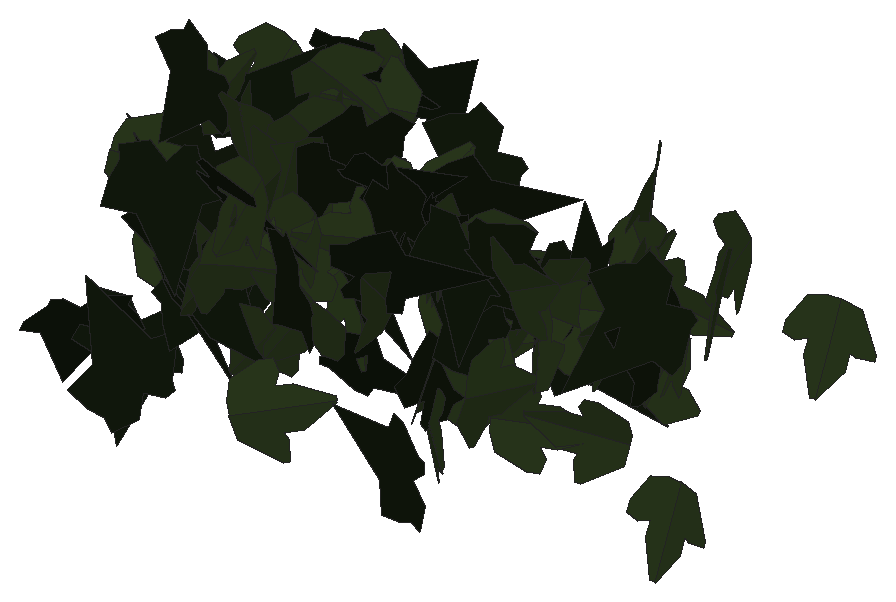
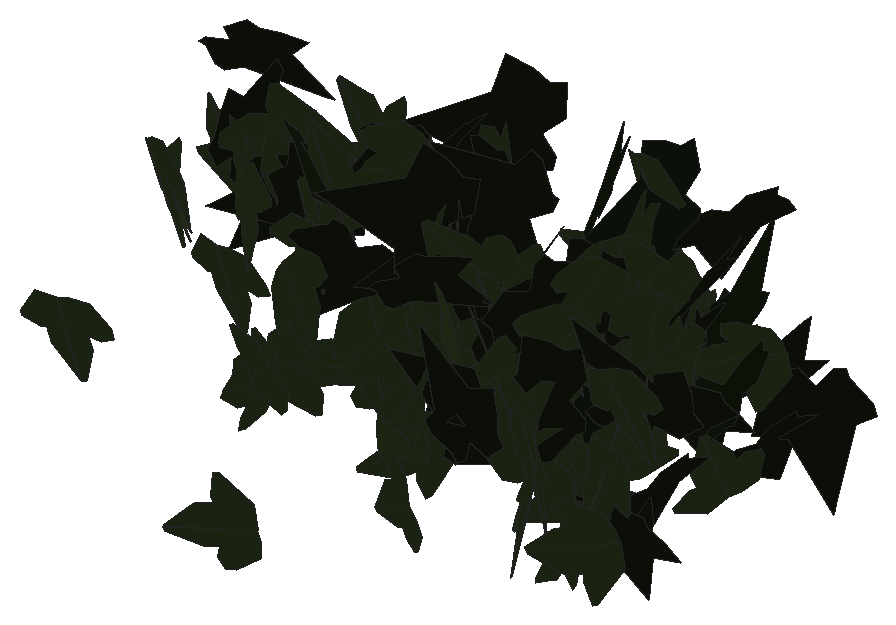
# SketchUp Ruby script. Lengths in inches.
U = 1.inch
M = Sketchup.active_model
def pt(a) = Geom::Point3d.new(a.map { |v| v * U })
def face(e, loops, mat)
  f = e.add_face(loops[0].map { |a| pt(a) })
  loops[1..].each { |l| e.add_face(l.map { |a| pt(a) }).erase! }
  f.material = f.back_material = mat if mat
  f
end
# faces: each face lists its corners as indices into pts; further lists are holes
def faces(e, pts, list, mat = nil) = list.each { |f| face(e, (f[0].is_a?(Array) ? f : [f]).map { |l| l.map { |i| pts[i] } }, mat) }
# xy, xz, yz: faces in a plane at the given z, y or x. An outline is a flat list of corners, or four numbers for a rectangle; further outlines are holes
def ring(l) = l.size == 4 ? [[l[0], l[1]], [l[2], l[1]], [l[2], l[3]], [l[0], l[3]]] : l.each_slice(2).to_a
def flat(e, list, mat, &to3) = list.each { |f| face(e, (f[0].is_a?(Array) ? f : [f]).map { |l| ring(l).map { |u, v| to3.(u, v) } }, mat) }
def xy(e, z, list, mat = nil) = flat(e, list, mat) { |x, y| [x, y, z] }
def xz(e, y, list, mat = nil) = flat(e, list, mat) { |x, z| [x, y, z] }
def yz(e, x, list, mat = nil) = flat(e, list, mat) { |y, z| [x, y, z] }
def lines(e, pts, list) = list.each { |a, b| e.add_line(pt(pts[a]), pt(pts[b])) }
# prism: a flat outline (further loops are holes) pulled along v
def prism(e, loops, v, mat = nil)
  f = face(e, loops, mat); d = Geom::Vector3d.new(v.map { |x| x * U })
  f.pushpull(f.normal.samedirection?(d) ? d.length : -d.length)
end
def box(e, o, s, mat = nil) = prism(e, [[o, [o[0] + s[0], o[1], o[2]], [o[0] + s[0], o[1] + s[1], o[2]], [o[0], o[1] + s[1], o[2]]]], [0, 0, s[2]], mat)
def at(x, y, z, deg = 0) = Geom::Transformation.translation(pt([x, y, z])) * Geom::Transformation.rotation(ORIGIN, Z_AXIS, deg.degrees)
def axes(o, x, y, z) = Geom::Transformation.new([*x, 0, *y, 0, *z, 0, *pt(o).to_a, 1])
def part(name) = M.definitions.add(name)
# library, detail: a bought-in or finely detailed component or shape, given as its bounding box
def library(name, o, s) = part(name).tap { |d| box(d.entities, o, s) }
def detail(e, o, s) = box(e.add_group.entities, o, s)
def put(e, d, t, mat = nil) = e.add_instance(d, t).tap { |i| i.material = mat if mat }
def group(e, t, mat = nil) = e.add_group.tap { |g| g.transformation = t; g.material = mat if mat }.entities
root = M.entities
M.materials.add("efeu1").color = [18, 25, 13]
M.materials.add("efeu2").color = [43, 57, 29]
c1 = part("ivyleaf_9")
p = [[1.54,2.16,1.25],[1.36,2.04,1.19],[-0.21,0.99,0.68],[-0.71,1.11,0.82],[-0.85,0.86,0.67],[-0.8,0.17,0.21],
  [-0.9,-0.01,0.1],[-0.67,-0.16,-0.02],[-0.08,-0.08,-0.05],[-0.03,-0.6,-0.4],[0.65,-0.88,-0.66],[0.83,-0.6,-0.49],
  [1.29,-0.42,-0.43],[1.8125,-0.07,-0.26],[1.21,0.44,0.15]]
faces(c1.entities,p,[[0,1,2,3,4,5,6,7,8,9,10,11,12,13,14]],"efeu1")
c2 = part("ivyleaf_10")
p = [[0,0.5,-0.03],[-0.0625,2.02,-0.43],[-0.19,2.01,-0.46],[-0.54,1.05,-0.29],[-0.52,0.625,-0.18],[-0.83,0.76,-0.28],
  [-1.16,0.64,-0.33],[-1.15,0.33,-0.24],[-0.77,-0.39,0.02],[-0.3,-0.51,0.16],[0.04,-0.48,0.23],[-0.02,2.01,-0.4375],
  [-0.06,2.01,-0.43],[0.04,-0.49,0.23],[0.67,-0.49,0.14],[1.38,0.36,-0.2],[1.375,0.51,-0.24],[0.81,0.65,-0.19],
  [0.62,0.59,-0.15],[0.6,1.09,-0.28],[0.5,1.23,-0.31]]
faces(c2.entities,p,[[0,1,2,3,4,5,6,7,8,9,10],[11,12,0,13,14,15,16,17,18,19,20]],"efeu2")
put(root,c1,axes([525.73,135.11,155.54],[0.37666,-0.56346,0.39178],[0.22865,-0.31835,-0.67766],[0.64707,0.44048,0.0114]))
put(root,c2,axes([526.19,134.96,153.36],[0.33775,0.58636,-0.33865],[0.14241,0.30846,0.67612],[0.66198,-0.36552,0.02733]))
put(root,c1,axes([526.49,131.96,153.91],[0.23337,0.62056,-0.38436],[-0.13918,-0.3583,-0.66299],[-0.71657,0.2717,0.00359]))
put(root,c2,axes([526.46,137.81,156.6],[0.70776,-0.14583,-0.30515],[-0.29443,0.08256,-0.72236],[0.16641,0.7663,0.01975]))
put(root,c2,axes([526.28,135.94,156.4],[0.05117,0.19029,-0.67696],[0.14044,0.66231,0.19679],[0.68903,-0.14913,0.01016]))
put(root,c2,axes([525.83,134.31,155.91],[-0.14356,-0.14885,-0.75209],[0.73421,0.19361,-0.17847],[0.22074,-0.74078,0.10448]))
put(root,c2,axes([526.39,138.1,155.05],[-0.66717,0.22134,-0.14554],[0.13083,-0.06761,-0.70256],[-0.23034,-0.6795,0.0225]))
put(root,c1,axes([526.29,137.07,154.2],[-0.03514,-0.79581,0.03387],[0.00121,-0.03395,-0.79658],[0.79653,-0.03505,0.0027]))
put(root,c1,axes([526.53,135.75,155.45],[-0.62542,-0.36181,-0.31053],[0.26494,0.16212,-0.72251],[0.39641,-0.67919,-0.00704]))
put(root,c2,axes([526.84,137.6875,154.86],[0.05179,0.09369,-0.70529],[-0.46103,-0.5342,-0.10482],[-0.54191,0.46342,0.02177]))
put(root,c2,axes([526.11,138.74,153.84],[-0.30774,0.05623,-0.71935],[0.7176,-0.05784,-0.31151],[-0.07537,-0.78027,-0.02874]))
put(root,c2,axes([526.68,137.98,154.46],[-0.33118,0.62006,0.1589],[0.0703,-0.14259,0.70295],[0.63623,0.33852,0.00504]))
put(root,c1,axes([526.71,137.6875,153.73],[-0.71609,-0.28278,-0.3521],[0.32978,0.1235,-0.76988],[0.30852,-0.78836,0.00569]))
put(root,c2,axes([526.35,137.02,155.77],[0.23807,-0.32545,0.65801],[0.50385,-0.43064,-0.39529],[0.53388,0.55154,0.07963]))
put(root,c1,axes([526.59,135.45,157.38],[-0.12657,-0.54335,0.52327],[-0.05752,-0.52209,-0.55604],[0.75216,-0.13135,0.04553]))
put(root,c1,axes([526.41,136.85,155.47],[-0.35697,0.12119,0.75407],[0.71327,-0.24468,0.37698],[0.27305,0.79761,0.00107]))
put(root,c2,axes([527.42,137.72,153.65],[0.24405,-0.16605,-0.66016],[-0.53993,0.37987,-0.29515],[0.41456,0.5925,0.00422]))
put(root,c1,axes([526.87,133.15,153.21],[-0.14848,-0.76576,0.05285],[-0.01587,-0.05076,-0.78],[0.76742,-0.14921,-0.0059]))
put(root,c2,axes([527.35,139.04,155.32],[0.34899,-0.44864,-0.39026],[-0.20276,0.33561,-0.56713],[0.55899,0.40183,0.03794]))
put(root,c2,axes([527.43,138.9375,156.24],[-0.11381,-0.59526,0.33256],[-0.04662,-0.32958,-0.60588],[0.68026,-0.12218,0.01412]))
put(root,c2,axes([527.82,137.77,154.49],[-0.47095,-0.11357,0.54585],[-0.50765,-0.20807,-0.48128],[0.23051,-0.69025,0.05527]))
put(root,c2,axes([527.48,135.5,156.73],[-0.73484,0.04403,0.0393],[-0.03958,-0.00361,-0.73613],[-0.04377,-0.73588,0.00596]))
put(root,c2,axes([527.48,138.98,154.92],[-0.33483,0.53964,0.27175],[-0.17377,0.21156,-0.63421],[-0.57867,-0.37578,0.03321]))
put(root,c2,axes([527.47,137.78,153.18],[0.03047,-0.14897,-0.70715],[0.0189,0.7077,-0.14827],[0.72242,-0.01223,0.03371]))
put(root,c1,axes([527.23,136.64,152.72],[-0.34943,0.15803,0.67847],[0.41809,-0.55957,0.34567],[0.55722,0.51896,0.16611]))
put(root,c2,axes([527.51,139.19,155.31],[-0.59921,-0.22011,0.27285],[0.2718,0.04956,0.63688],[-0.22141,0.65654,0.0434]))
put(root,c1,axes([527.08,138.56,156.42],[0.66341,-0.03506,0.43888],[0.43733,-0.03928,-0.6642],[0.0509,0.79447,-0.01347]))
put(root,c2,axes([527.96,139.09,156.48],[0.50985,-0.29969,-0.37154],[-0.31309,0.20041,-0.59128],[0.36033,0.59818,0.01196]))
put(root,c2,axes([528.09,136.21,153.87],[0.43176,-0.20389,0.53418],[-0.48313,0.2279,0.47748],[-0.30579,-0.64795,-0.00015]))
put(root,c1,axes([527.68,132.93,155.23],[0.55391,-0.54398,-0.11808],[0.08585,-0.08111,0.77635],[-0.54999,-0.56052,0.00226]))
put(root,c1,axes([528.06,136.39,155.44],[-0.3816,0.41646,-0.52655],[0.36418,-0.3804,-0.56479],[-0.56398,-0.52742,-0.00842]))
put(root,c1,axes([528.27,131.45,153.125],[-0.46136,-0.60384,0.18477],[0.11557,0.14422,0.75991],[-0.62081,0.4756,0.00415]))
put(root,c2,axes([528.04,137.41,156.07],[-0.06281,-0.44523,-0.52849],[0.05937,0.52523,-0.44954],[0.68848,-0.08591,-0.00945]))
put(root,c2,axes([527.63,136.95,153.6],[0.15666,0.15875,0.68166],[0.39485,0.5567,-0.22039],[-0.57788,0.42341,0.0342]))
put(root,c2,axes([527.87,137.4,157],[-0.51535,-0.23976,-0.514],[0.47284,0.20192,-0.56826],[0.31323,-0.69929,0.01215]))
put(root,c2,axes([528.47,137.875,153.66],[-0.3783,0.42346,0.46618],[-0.30882,0.34922,-0.56783],[-0.54888,-0.48835,-0.00182]))
put(root,c1,axes([528.1,132.43,157.25],[-0.11932,-0.75762,-0.22579],[0.02574,0.22451,-0.76691],[0.79013,-0.12173,-0.00912]))
put(root,c2,axes([528.26,136.81,154.4],[0.61908,0.36942,0.04018],[0.03531,0.01923,-0.72092],[-0.36992,0.62009,-0.00157]))
put(root,c2,axes([528.75,138.28,156.12],[0.13292,0.19344,0.65385],[-0.33366,-0.5625,0.23424],[0.59465,-0.35886,-0.01471]))
put(root,c2,axes([527.94,135.1,154.68],[0.35602,0.15154,0.64477],[0.5863,0.26844,-0.38682],[-0.30813,0.68587,0.00894]))
put(root,c2,axes([528.44,136.35,155.38],[0.05455,0.30482,-0.67747],[-0.08227,-0.67264,-0.30927],[-0.73832,0.09747,-0.01559]))
put(root,c2,axes([528.41,133.25,154.74],[-0.0758,0.11365,0.83409],[0.47877,-0.68301,0.13657],[0.69239,0.48472,-0.00312]))
put(root,c1,axes([528.17,132.82,154.48],[0.45781,-0.56256,0.32268],[0.20926,-0.24572,-0.72527],[0.61385,0.50332,0.00658]))
put(root,c1,axes([528.57,132.77,155],[0.16251,-0.46561,-0.62034],[-0.12427,0.60999,-0.4904],[0.76562,0.19784,0.05207]))
put(root,c2,axes([528.71,135.53,157.05],[-0.37942,-0.41519,-0.37968],[0.26265,0.27427,-0.5624],[0.49755,-0.4614,0.00735]))
put(root,c1,axes([528.65,139.36,155.46],[-0.24925,0.09443,0.71655],[0.50871,-0.51549,0.24489],[0.51339,0.55664,0.10522]))
put(root,c2,axes([529.16,134.7,156.82],[-0.28766,-0.75884,0.09762],[-0.02405,-0.09528,-0.81145],[0.76471,-0.28844,0.01121]))
put(root,c2,axes([529.62,133.51,153.81],[-0.54475,-0.1323,0.46695],[-0.45395,-0.10941,-0.56059],[0.17168,-0.70911,-0.00062]))
put(root,c2,axes([529.07,132.65,155.52],[-0.18011,-0.28273,-0.72286],[0.38507,0.61176,-0.33523],[0.67393,-0.42511,-0.00165]))
put(root,c1,axes([529.54,136.37,156.77],[-0.09222,0.37815,-0.77973],[0.16906,-0.76122,-0.38917],[-0.84994,-0.19245,0.00719]))
put(root,c2,axes([529.18,133.98,156.65],[-0.0628,0.07664,0.88256],[0.4505,-0.75907,0.09797],[0.76278,0.45462,0.0148]))
put(root,c1,axes([529.02,134.82,156.35],[0.18557,0.30961,-0.69755],[0.35331,0.60146,0.36095],[0.67647,-0.39907,0.00284]))
put(root,c2,axes([529.02,137.51,155.06],[-0.00553,0.02222,-0.80273],[0.64831,-0.47358,-0.01758],[-0.47388,-0.64817,-0.01467]))
put(root,c2,axes([529.8,134.24,155.79],[0.64503,-0.3477,-0.28676],[-0.252,0.13685,-0.73278],[0.37366,0.69251,0.00083]))
put(root,c1,axes([529.2,132.51,157.28],[0.78111,-0.2162,0.19855],[0.19335,-0.04571,-0.81045],[0.22086,0.80465,0.00731]))
put(root,c2,axes([529.39,134.41,154.76],[0.43202,0.20004,-0.62224],[0.53966,0.31162,0.47487],[0.36873,-0.69045,0.03404]))
put(root,c2,axes([530.04,132.39,157.39],[0.67732,-0.3914,-0.31063],[-0.26731,0.15825,-0.78227],[0.42217,0.72816,0.00304]))
put(root,c2,axes([530.63,133.37,154.72],[-0.68411,-0.16117,0.54079],[-0.529,-0.11269,-0.70278],[0.19644,-0.86473,-0.00921]))
put(root,c1,axes([530.7,136.16,154.95],[-0.06331,0.2723,0.7111],[-0.24205,0.66935,-0.27786],[-0.72196,-0.24829,0.0308]))
put(root,c1,axes([529.63,137.25,154.41],[0.19437,-0.07367,0.84761],[0.77775,-0.33712,-0.20765],[0.34494,0.80161,-0.00942]))
put(root,c2,axes([530.97,134.86,155.7],[0.05622,0.03281,0.71911],[-0.49015,-0.52652,0.06235],[0.52721,-0.49301,-0.01873]))
put(root,c2,axes([530.9,135.92,156.15],[0.46301,-0.39093,-0.41607],[-0.3309,0.25279,-0.60574],[0.46524,0.56885,-0.01676]))
put(root,c2,axes([530.15,139.28,153.46],[0.32042,-0.11567,0.69432],[0.67291,-0.17348,-0.33944],[0.20651,0.74475,0.02877]))
put(root,c1,axes([530.57,134.89,155.03],[0.56537,-0.36927,-0.42469],[-0.35413,0.23445,-0.67528],[0.4374,0.66712,0.00223]))
put(root,c2,axes([530.53,134.81,154.58],[0.58943,-0.1697,0.4472],[0.42898,-0.12637,-0.61337],[0.21158,0.72901,-0.00222]))
put(root,c2,axes([531.11,137.57,154.77],[0.05845,0.15944,-0.73633],[-0.1167,0.73154,0.14914],[0.7443,0.10218,0.08121]))
put(root,c1,axes([530.59,134.36,153.34],[0.63359,-0.06482,0.47014],[0.46697,-0.05472,-0.63687],[0.08464,0.78706,-0.00556]))
put(root,c1,axes([531.84,137.23,156.71],[-0.55919,-0.43601,0.27616],[-0.2196,-0.16748,-0.70908],[0.46706,-0.60076,-0.00275]))
put(root,c2,axes([531.48,136.34,155.3],[0.5336,-0.55502,-0.01206],[0.01156,-0.00561,0.76991],[-0.55503,-0.53371,0.00445]))
put(root,c1,axes([531.4,132.12,156.05],[-0.03624,-0.32301,0.75298],[0.05393,-0.75302,-0.32043],[0.81756,0.03535,0.05452]))
put(root,c2,axes([531.43,135.43,156.14],[0.5123,0.32592,-0.55248],[0.45205,0.3182,0.60689],[0.45509,-0.68296,0.0191]))
put(root,c1,axes([531.22,134.5,157.02],[0.58662,0.32956,-0.39131],[0.32535,0.21914,0.67229],[0.39482,-0.67024,0.0274]))
put(root,c2,axes([531.79,137.67,153.91],[0.17378,-0.53167,0.51439],[0.15306,-0.49112,-0.55933],[0.72377,0.23152,-0.00523]))
put(root,c2,axes([532.12,135.99,154.32],[0.61286,-0.05358,0.41692],[-0.41608,0.02749,0.61515],[-0.05977,-0.74072,-0.00733]))
put(root,c1,axes([531.96,134.64,155.94],[0.15705,0.21496,0.73889],[0.24435,0.70116,-0.25592],[-0.7297,0.28106,0.07333]))
put(root,c2,axes([531.73,136.44,153.02],[-0.03118,-0.14763,-0.75567],[0.48735,0.58172,-0.13375],[0.59609,-0.48333,0.06983]))
put(root,c2,axes([531.51,130.67,154.16],[0.20551,0.02166,-0.78165],[0.7732,0.11491,0.20648],[0.11663,-0.8,0.0085]))
put(root,c1,axes([531.92,134.18,157.22],[-0.05725,-0.04436,-0.82621],[0.79741,0.21799,-0.06695],[0.22074,-0.79898,0.0276]))
put(root,c1,axes([532.14,134.64,155.95],[0.54878,0.22463,0.5522],[0.50604,0.22122,-0.59289],[-0.31513,0.74642,0.00954]))
put(root,c2,axes([532.49,135.35,156.35],[0.14707,-0.39968,0.69972],[0.40955,-0.57549,-0.4148],[0.69399,0.42432,0.09651]))
put(root,c2,axes([532.72,136.26,154.72],[-0.00258,-0.06448,-0.77656],[0.19562,0.75164,-0.06306],[0.75427,-0.19516,0.0137]))
put(root,c2,axes([532.96,136.34,154.09],[-0.10456,-0.43135,0.57598],[-0.11579,-0.56436,-0.44367],[0.71021,-0.15551,0.01247]))
put(root,c2,axes([532.77,134.19,153.42],[0.32285,-0.76799,0.1296],[-0.04993,0.1196,0.83309],[-0.77724,-0.32669,0.00031]))
put(root,c2,axes([532.82,134.96,154.35],[0.76639,0.1115,0.03958],[-0.03917,-0.00567,0.77445],[0.11164,-0.76739,0.00002]))
put(root,c1,axes([532.72,134.27,153.28],[0.00662,0.03793,0.80643],[0.55066,0.58952,-0.03225],[-0.59037,0.5503,-0.02103]))
put(root,c2,axes([533.24,136.39,155.03],[-0.43748,-0.56914,0.1306],[-0.07998,-0.10325,-0.71785],[0.57843,-0.44473,-0.00048]))
put(root,c2,axes([532.7,134.41,152.7],[-0.07548,0.06886,-0.76785],[0.41704,-0.64524,-0.09886],[-0.64839,-0.42303,0.02579]))
put(root,c1,axes([532.51,135.27,156.77],[0.36655,-0.00786,0.73551],[0.73501,0.03547,-0.36592],[-0.02825,0.82102,0.02286]))
put(root,c2,axes([532.75,134.43,156.38],[0.06314,-0.03133,0.7733],[0.62401,-0.45689,-0.06946],[0.45781,0.62708,-0.01198]))
put(root,c2,axes([533.31,132.45,156.24],[-0.11521,-0.55365,-0.58018],[-0.04052,-0.58136,0.56283],[-0.80093,0.10906,0.05498]))
put(root,c2,axes([533.54,135.1,153.28],[-0.01385,0.59627,0.47066],[-0.02094,-0.47086,0.5959],[0.75935,-0.00211,0.02501]))
put(root,c2,axes([532.91,140.65,152.62],[0.138,0.01796,0.76106],[0.69454,0.31373,-0.13335],[-0.31171,0.70699,0.03983]))
put(root,c1,axes([533.8,132.37,152.79],[0.15673,-0.79501,0.05984],[0.0044,0.06185,0.81015],[-0.79725,-0.15595,0.01623]))
put(root,c1,axes([533.07,131.87,156.97],[0.45293,0.05067,0.6925],[0.6848,0.10406,-0.45551],[-0.11477,0.82089,0.01499]))
put(root,c1,axes([534.01,134.28,155],[-0.1225,-0.79978,0.1421],[0.02146,0.14047,0.80911],[-0.81202,0.12436,-0.00006]))
put(root,c2,axes([534.17,138.42,154.25],[0.11963,-0.23907,0.6877],[-0.2474,0.6421,0.26625],[-0.68474,-0.27376,0.02394]))
put(root,c1,axes([533.87,133.92,156.98],[0.03729,-0.79551,0.19246],[0.0098,-0.19221,-0.79638],[0.8184,0.03855,0.00076]))
put(root,c2,axes([533.7,138.98,154.92],[0.49195,-0.01391,0.55242],[0.55161,-0.0318,-0.49203],[0.03299,0.73904,-0.01077]))
put(root,c2,axes([534.07,134.21,157.15],[-0.56963,-0.02773,-0.54153],[0.54063,0.03134,-0.57029],[0.04169,-0.78533,-0.00364]))
put(root,c1,axes([534.06,133.92,156.89],[0.01674,-0.05946,-0.84196],[0.41918,0.73152,-0.04333],[0.73261,-0.4172,0.04403]))
put(root,c1,axes([534.21,135.7,155.78],[-0.2649,-0.3171,-0.72918],[0.46867,0.55862,-0.41319],[0.64235,-0.53835,0.00076]))
put(root,c2,axes([534.18,134.88,152.97],[0.01203,-0.00891,0.78498],[0.59417,0.5132,-0.00329],[-0.51307,0.59411,0.01461]))
put(root,c2,axes([534.89,136.68,155.33],[0.07488,-0.75365,0.13839],[0.01684,-0.1374,-0.75736],[0.76607,0.07668,0.00312]))
put(root,c2,axes([535.78,135.64,152.85],[-0.18191,0.03462,-0.74937],[-0.73067,-0.18282,0.16892],[-0.16991,0.74914,0.07585]))
put(root,c2,axes([535.42,137.36,157.46],[0.19391,-0.66201,-0.33805],[-0.09624,0.32407,-0.68983],[0.73707,0.21648,-0.00113]))
put(root,c2,axes([535.17,135.58,155.68],[0.75039,0.13199,0.07397],[0.07202,0.01753,-0.7619],[-0.13307,0.75382,0.00477]))
put(root,c2,axes([535.24,134.82,155.91],[-0.69572,-0.09009,0.43905],[0.44077,0.0095,0.70039],[-0.08128,0.82262,0.04]))
put(root,c2,axes([535.84,135.04,155.92],[0.38424,-0.50992,-0.53406],[-0.30507,0.43863,-0.6383],[0.67244,0.49038,0.01559]))
put(root,c1,axes([536.09,134.47,156.36],[-0.61872,0.31415,-0.51079],[-0.45628,0.22961,0.69391],[0.38912,0.76877,0.00148]))
put(root,c2,axes([535.21,133.68,156.58],[-0.46983,-0.01352,0.68213],[0.68053,-0.0684,0.46737],[0.0487,0.82545,0.04991]))
put(root,c2,axes([536.01,133.42,155.35],[0.55929,-0.32441,0.39513],[-0.33416,0.21125,0.64644],[-0.38692,-0.65138,0.01286]))
put(root,c2,axes([535.82,131.8125,155.53],[-0.04435,-0.2532,-0.78851],[0.20905,0.76065,-0.25601],[0.80135,-0.21245,0.02315]))
put(root,c1,axes([535.8,134.38,155.86],[0.25281,0.19222,-0.71859],[0.25415,0.69096,0.27424],[0.69908,-0.32071,0.16016]))
put(root,c2,axes([535.96,134,156.08],[0.11648,0.01211,0.80753],[0.70146,0.40282,-0.10722],[-0.40024,0.70951,0.0471]))
put(root,c1,axes([536.33,134.34,155.88],[-0.12657,-0.23034,-0.74412],[0.37681,0.64169,-0.26273],[0.68175,-0.39744,0.00707]))
put(root,c2,axes([536.76,134.67,155.88],[-0.06659,-0.29974,-0.72216],[-0.02345,-0.72368,0.30253],[-0.78154,0.04726,0.05245]))
put(root,c2,axes([536.87,134.1,156.54],[0.05007,-0.00593,0.74554],[0.48583,0.56705,-0.02811],[-0.56554,0.4866,0.04185]))
put(root,c2,axes([537.8,136.93,156.97],[0.52554,-0.45018,-0.41172],[-0.29648,0.28648,-0.69167],[0.53318,0.60303,0.02122]))
put(root,c2,axes([537.53,136.79,156.49],[0.45398,-0.50056,0.41985],[0.28462,-0.30867,-0.67576],[0.58808,0.53581,0.00294]))
put(root,c1,axes([538.06,134.41,155.95],[0.03784,0.05672,0.78925],[-0.36356,-0.70056,0.06778],[0.70282,-0.36545,-0.00743]))
put(root,c2,axes([538.26,134.39,156.36],[0.65641,-0.40807,-0.18808],[-0.1612,0.09692,-0.77291],[0.41941,0.67591,-0.00272]))
put(root,c2,axes([538.19,139.18,154.65],[0.7647,0.07383,-0.06299],[-0.06264,-0.00663,-0.76825],[-0.07413,0.76726,-0.00058]))
put(root,c2,axes([538.08,134.25,155.36],[0.7196,-0.28767,-0.24903],[0.2308,-0.09352,0.77497],[-0.30249,-0.75571,-0.00111]))
put(root,c1,axes([538.72,133.53,157.59],[-0.74783,-0.29792,0.1534],[-0.1426,-0.05653,-0.80499],[0.30324,-0.76131,-0.00026]))
put(root,c2,axes([538.61,133.97,153.28],[0.76675,-0.11645,-0.02617],[-0.02543,0.00684,-0.77554],[0.11661,0.76716,0.00294]))
